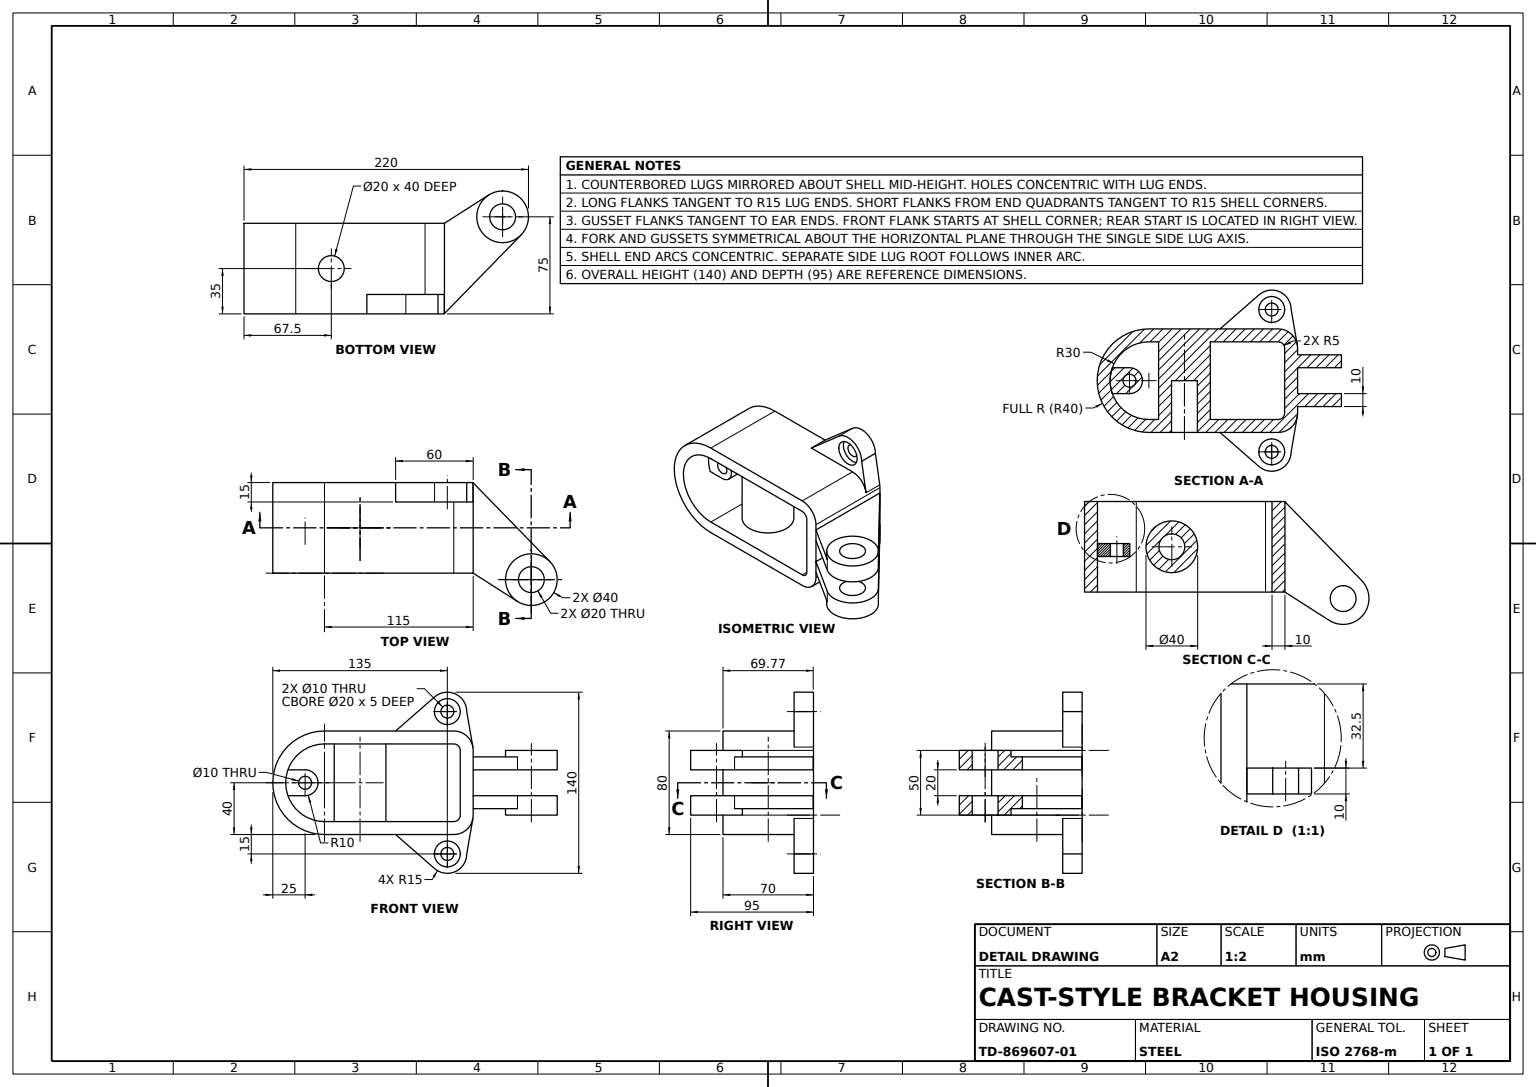
solid
v1 (70,-40,0)
v2 (15,-40,0)
e1 v1 v2 LINE
v3 (-25,0,0)
e2 v3 v2 CIRCLE(AX(P(15,0,0),D(0,0,1),D(1,0,0)),40)
v4 (15,40,0)
e3 v4 v3 CIRCLE(AX(P(15,0,0),D(0,0,1),D(1,0,0)),40)
v5 (70,40,0)
e4 v4 v5 LINE
v6 (100.136986,66.30137,0)
e5 v6 v5 LINE
v7 (125,55,0)
e6 v7 v6 CIRCLE(AX(P(110,55,0),D(0,0,1),D(1,0,0)),15)
v8 (129.77747,27.574177,0)
e7 v7 v8 LINE
v9 (130,25,0)
e8 v8 v9 CIRCLE(AX(P(115,25,0),D(0,0,-1),D(1,0,0)),15)
v10 (130,-25,0)
e9 v9 v10 LINE
v11 (129.77747,-27.574177,0)
e10 v10 v11 CIRCLE(AX(P(115,-25,0),D(0,0,-1),D(1,0,0)),15)
v12 (125,-55,0)
e11 v12 v11 LINE
v13 (100.136986,-66.30137,0)
e12 v12 v13 CIRCLE(AX(P(110,-55,0),D(0,0,-1),D(1,0,0)),15)
e13 v13 v1 LINE
v14 (105,55,0)
v15 (115,55,0)
e14 v14 v15 CIRCLE(AX(P(110,55,0),D(0,0,1),D(1,0,0)),5)
e15 v15 v14 CIRCLE(AX(P(110,55,0),D(0,0,1),D(1,0,0)),5)
v16 (120,25,0)
v17 (120,-25,0)
e16 v16 v17 LINE
v18 (115,30,0)
e17 v18 v16 CIRCLE(AX(P(115,25,0),D(0,0,-1),D(1,0,0)),5)
v19 (15,30,0)
e18 v19 v18 LINE
v20 (-15,0,0)
e19 v19 v20 CIRCLE(AX(P(15,0,0),D(0,0,1),D(1,0,0)),30)
v21 (15,-30,0)
e20 v20 v21 CIRCLE(AX(P(15,0,0),D(0,0,1),D(1,0,0)),30)
v22 (115,-30,0)
e21 v22 v21 LINE
e22 v17 v22 CIRCLE(AX(P(115,-25,0),D(0,0,-1),D(1,0,0)),5)
v23 (115,-55,0)
v24 (105,-55,0)
e23 v23 v24 CIRCLE(AX(P(110,-55,0),D(0,0,-1),D(1,0,0)),5)
e24 v24 v23 CIRCLE(AX(P(110,-55,0),D(0,0,-1),D(1,0,0)),5)
face PLANE(AX(P(0,0,0),D(0,0,1),D(1,0,0))) rev [e1 -e2 -e3 e4 -e5 -e6 e7 e8 e9 e10 -e11 e12 e13] [e14 e15] [-e16 -e17 -e18 e19 e20 -e21 -e22] [-e23 -e24]
v25 (100,55,15)
v26 (120,55,15)
e25 v25 v26 CIRCLE(AX(P(110,55,15),D(0,0,1),D(1,0,0)),10)
v27 (120,55,10)
e26 v26 v27 LINE
v28 (100,55,10)
e27 v28 v27 CIRCLE(AX(P(110,55,10),D(0,0,1),D(1,0,0)),10)
e28 v25 v28 LINE
face CYL(AX(P(110,55,15),D(0,0,-1),D(-1,0,0)),10) rev [e25 e26 -e27 -e28]
v29 (42.5,30,55)
v30 (42.5,30,15)
e29 v29 v30 CIRCLE(AX(P(42.5,30,35),D(0,-1,0),D(0,0,1)),20)
v31 (42.5,-30,15)
e30 v30 v31 LINE
v32 (42.5,-30,55)
e31 v31 v32 CIRCLE(AX(P(42.5,-30,35),D(0,1,0),D(0,0,-1)),20)
e32 v29 v32 LINE
face CYL(AX(P(42.5,86.568542,35),D(0,-1,0),D(0,0,-1)),20) [e29 e30 e31 -e32]
v33 (130,-25,70)
v34 (115,-40,70)
e33 v33 v34 CIRCLE(AX(P(115,-25,70),D(0,0,-1),D(1,0,0)),15)
v35 (115,-40,15)
e34 v34 v35 LINE
v36 (129.77747,-27.574177,15)
e35 v36 v35 CIRCLE(AX(P(115,-25,15),D(0,0,-1),D(1,0,0)),15)
e36 v36 v11 LINE
e37 v33 v10 LINE
face CYL(AX(P(115,-25,70),D(0,0,-1),D(-1,0,0)),15) [e33 e34 -e35 e36 -e10 -e37]
v37 (189.316428,-10,61.034332)
v38 (130,-10,0.228119)
e38 v37 v38 LINE
v39 (189.316428,-20,61.034332)
e39 v39 v37 LINE
v40 (130,-20,0.228119)
e40 v39 v40 LINE
e41 v40 v38 LINE
face PLANE(AX(P(66.498013,-20,-64.868776),D(0.715821408,0,-0.698283403),D(-0.698283403,0,-0.715821408))) [-e38 -e39 e40 e41]
v41 (175,25,55)
v42 (175,25,95)
e42 v41 v42 CIRCLE(AX(P(175,25,75),D(0,1,0),D(0,0,1)),20)
v43 (175,20,55)
e43 v41 v43 LINE
v44 (164.238039,20,91.857645)
e44 v43 v44 CIRCLE(AX(P(175,20,75),D(0,1,0),D(0,0,1)),20)
v45 (164.238039,10,91.857645)
e45 v44 v45 LINE
v46 (175,10,95)
e46 v45 v46 CIRCLE(AX(P(175,10,75),D(0,1,0),D(0,0,1)),20)
e47 v42 v46 LINE
face CYL(AX(P(175,25,75),D(0,-1,0),D(0,0,-1)),20) [-e42 e43 e44 e45 e46 -e47]
e48 v42 v41 CIRCLE(AX(P(175,25,75),D(0,1,0),D(0,0,1)),20)
v47 (175,25,85)
v48 (175,25,65)
e49 v47 v48 CIRCLE(AX(P(175,25,75),D(0,1,0),D(0,0,1)),10)
e50 v48 v47 CIRCLE(AX(P(175,25,75),D(0,1,0),D(0,0,1)),10)
face PLANE(AX(P(0,25,0),D(0,1,0),D(0,0,1))) [e48 e42] [-e49 -e50]
v49 (100,-55,15)
v50 (100,-55,10)
e51 v49 v50 LINE
v51 (120,-55,15)
e52 v51 v49 CIRCLE(AX(P(110,-55,15),D(0,0,-1),D(1,0,0)),10)
v52 (120,-55,10)
e53 v51 v52 LINE
e54 v52 v50 CIRCLE(AX(P(110,-55,10),D(0,0,-1),D(1,0,0)),10)
face CYL(AX(P(110,-55,15),D(0,0,-1),D(-1,0,0)),10) rev [-e51 -e52 e53 e54]
v53 (105,-55,10)
e55 v53 v24 LINE
v54 (115,-55,10)
e56 v54 v23 LINE
e57 v54 v53 CIRCLE(AX(P(110,-55,10),D(0,0,1),D(1,0,0)),5)
face CYL(AX(P(110,-55,70),D(0,0,-1),D(-1,0,0)),5) rev [e55 e24 -e56 e57]
v55 (-15,0,70)
e58 v55 v20 LINE
v56 (15,-30,70)
e59 v55 v56 CIRCLE(AX(P(15,0,70),D(0,0,1),D(1,0,0)),30)
e60 v56 v21 LINE
face CYL(AX(P(15,0,70),D(0,0,-1),D(-1,0,0)),30) rev [-e20 -e58 e59 e60]
v57 (129.77747,27.574177,15)
e61 v57 v8 LINE
v58 (115,40,15)
e62 v58 v57 CIRCLE(AX(P(115,25,15),D(0,0,-1),D(1,0,0)),15)
v59 (115,40,70)
e63 v59 v58 LINE
v60 (130,25,70)
e64 v59 v60 CIRCLE(AX(P(115,25,70),D(0,0,-1),D(1,0,0)),15)
e65 v60 v9 LINE
face CYL(AX(P(115,25,70),D(0,0,-1),D(-1,0,0)),15) [-e61 -e62 -e63 e64 e65 -e8]
v61 (42.5,0,25)
v62 (42.5,0,45)
e66 v61 v62 CIRCLE(AX(P(42.5,0,35),D(0,1,0),D(0,0,1)),10)
e67 v62 v61 CIRCLE(AX(P(42.5,0,35),D(0,1,0),D(0,0,1)),10)
face PLANE(AX(P(0,0,0),D(0,1,0),D(0,0,1))) rev [-e66 -e67]
v63 (105,55,10)
e68 v63 v14 LINE
v64 (115,55,10)
e69 v64 v63 CIRCLE(AX(P(110,55,10),D(0,0,-1),D(1,0,0)),5)
e70 v64 v15 LINE
face CYL(AX(P(110,55,70),D(0,0,-1),D(-1,0,0)),5) rev [-e14 -e68 -e69 e70]
v65 (125,-55,15)
e71 v65 v36 LINE
e72 v65 v12 LINE
face PLANE(AX(P(130.617297,-22.753016,15),D(-0.985164654,0.171611782,0),D(-0.171611782,-0.985164654,0))) rev [-e36 -e71 e72 e11]
v66 (70,-40,15)
e73 v66 v1 LINE
v67 (100.136986,-66.30137,15)
e74 v67 v13 LINE
e75 v67 v66 LINE
face PLANE(AX(P(10.448489,11.972227,15),D(-0.657534247,-0.753424658,0),D(0.753424658,-0.657534247,0))) [e73 -e13 -e74 e75]
e76 v26 v25 CIRCLE(AX(P(110,55,15),D(0,0,1),D(1,0,0)),10)
v68 (100.136986,66.30137,15)
v69 (70,40,15)
e77 v68 v69 LINE
e78 v69 v58 LINE
v70 (125,55,15)
e79 v70 v57 LINE
e80 v70 v68 CIRCLE(AX(P(110,55,15),D(0,0,1),D(1,0,0)),15)
face PLANE(AX(P(0,0,15),D(0,0,1),D(1,0,0))) [-e25 -e76] [e77 e78 e62 -e79 e80]
v71 (42.5,-40,45)
e81 v71 v62 LINE
v72 (42.5,-40,25)
e82 v72 v61 LINE
e83 v72 v71 CIRCLE(AX(P(42.5,-40,35),D(0,-1,0),D(0,0,-1)),10)
face CYL(AX(P(42.5,-86.568542,35),D(0,1,0),D(0,0,1)),10) rev [e81 e67 -e82 e83]
v73 (175,10,85)
v74 (175,10,65)
e84 v73 v74 CIRCLE(AX(P(175,10,75),D(0,1,0),D(0,0,1)),10)
e85 v74 v73 CIRCLE(AX(P(175,10,75),D(0,1,0),D(0,0,1)),10)
v75 (189.316428,10,61.034332)
v76 (130,10,0.228119)
e86 v75 v76 LINE
e87 v46 v75 CIRCLE(AX(P(175,10,75),D(0,1,0),D(0,0,1)),20)
v77 (130,10,70)
e88 v45 v77 LINE
e89 v76 v77 LINE
face PLANE(AX(P(0,10,0),D(0,1,0),D(0,0,1))) rev [e84 e85] [-e86 -e87 -e46 e88 -e89]
v78 (115,-30,70)
e90 v78 v22 LINE
v79 (120,-25,70)
e91 v79 v78 CIRCLE(AX(P(115,-25,70),D(0,0,-1),D(1,0,0)),5)
e92 v79 v17 LINE
face CYL(AX(P(115,-25,70),D(0,0,-1),D(-1,0,0)),5) rev [-e90 -e91 e92 e22]
v80 (189.316428,20,61.034332)
e93 v80 v75 LINE
e94 v80 v43 CIRCLE(AX(P(175,20,75),D(0,1,0),D(0,0,1)),20)
face CYL(AX(P(175,25,75),D(0,-1,0),D(0,0,-1)),20) [e87 -e93 e94 -e43 -e48 e47]
e95 v27 v28 CIRCLE(AX(P(110,55,10),D(0,0,1),D(1,0,0)),10)
face CYL(AX(P(110,55,15),D(0,0,-1),D(-1,0,0)),10) rev [e28 -e95 -e26 e76]
v81 (-25,0,70)
e96 v81 v3 LINE
v82 (15,-40,70)
e97 v82 v2 LINE
e98 v81 v82 CIRCLE(AX(P(15,0,70),D(0,0,1),D(1,0,0)),40)
face CYL(AX(P(15,0,70),D(0,0,-1),D(-1,0,0)),40) [e96 e2 -e97 -e98]
v83 (164.238039,-10,91.857645)
v84 (130,-10,70)
e99 v83 v84 LINE
v85 (130,-20,70)
e100 v85 v84 LINE
v86 (164.238039,-20,91.857645)
e101 v86 v85 LINE
e102 v86 v83 LINE
face PLANE(AX(P(5.892704,-20,-9.230391),D(0.538098029,0,-0.842882264),D(-0.842882264,0,-0.538098029))) rev [e99 -e100 -e101 e102]
e103 v71 v72 CIRCLE(AX(P(42.5,-40,35),D(0,-1,0),D(0,0,-1)),10)
face CYL(AX(P(42.5,-86.568542,35),D(0,1,0),D(0,0,1)),10) rev [-e81 e103 e82 e66]
v87 (120,25,70)
e104 v87 v79 LINE
e105 v87 v16 LINE
face PLANE(AX(P(120,0,70),D(1,0,0),D(0,0,-1))) rev [e16 -e92 -e104 e105]
e106 v49 v51 CIRCLE(AX(P(110,-55,15),D(0,0,-1),D(1,0,0)),10)
e107 v50 v52 CIRCLE(AX(P(110,-55,10),D(0,0,-1),D(1,0,0)),10)
face CYL(AX(P(110,-55,15),D(0,0,-1),D(-1,0,0)),10) rev [-e106 e51 e107 -e53]
e108 v35 v66 LINE
e109 v34 v82 LINE
face PLANE(AX(P(0,-40,70),D(0,-1,0),D(1,0,0))) [-e103 -e83] [-e1 -e73 -e108 -e34 e109 e97]
v88 (15,40,70)
e110 v88 v59 LINE
e111 v69 v5 LINE
e112 v88 v4 LINE
face PLANE(AX(P(0,40,70),D(0,1,0),D(-1,0,0))) [e110 e63 -e78 e111 -e4 -e112]
e113 v65 v67 CIRCLE(AX(P(110,-55,15),D(0,0,-1),D(1,0,0)),15)
face CYL(AX(P(110,-55,15),D(0,0,-1),D(-1,0,0)),15) [e113 e74 -e12 -e72]
e114 v78 v56 LINE
e115 v32 v31 CIRCLE(AX(P(42.5,-30,35),D(0,1,0),D(0,0,-1)),20)
face PLANE(AX(P(0,-30,70),D(0,-1,0),D(0,0,-1))) rev [e21 -e60 -e114 e90] [-e31 -e115]
v89 (175,-25,85)
v90 (175,-10,85)
e116 v89 v90 LINE
v91 (175,-25,65)
e117 v91 v89 CIRCLE(AX(P(175,-25,75),D(0,1,0),D(0,0,1)),10)
v92 (175,-10,65)
e118 v91 v92 LINE
e119 v92 v90 CIRCLE(AX(P(175,-10,75),D(0,1,0),D(0,0,1)),10)
face CYL(AX(P(175,-25,75),D(0,1,0),D(0,0,1)),10) rev [-e116 -e117 e118 e119]
v93 (175,-25,55)
v94 (175,-20,55)
e120 v93 v94 LINE
v95 (175,-25,95)
e121 v93 v95 CIRCLE(AX(P(175,-25,75),D(0,1,0),D(0,0,1)),20)
v96 (175,-10,95)
e122 v95 v96 LINE
e123 v83 v96 CIRCLE(AX(P(175,-10,75),D(0,1,0),D(0,0,1)),20)
e124 v94 v86 CIRCLE(AX(P(175,-20,75),D(0,1,0),D(0,0,1)),20)
face CYL(AX(P(175,-25,75),D(0,1,0),D(0,0,1)),20) [-e120 e121 e122 -e123 -e102 -e124]
v97 (130,20,0.228119)
e125 v80 v97 LINE
v98 (130,20,70)
e126 v97 v98 LINE
e127 v44 v98 LINE
face PLANE(AX(P(0,20,0),D(0,1,0),D(0,0,1))) [-e44 -e94 e125 e126 -e127]
e128 v85 v40 LINE
e129 v85 v33 LINE
e130 v60 v98 LINE
e131 v97 v76 LINE
e132 v77 v84 LINE
e133 v84 v38 LINE
face PLANE(AX(P(130,0,70),D(1,0,0),D(0,0,-1))) [-e128 e129 e37 -e9 -e65 e130 -e126 e131 e89 e132 e133 -e41]
e134 v90 v92 CIRCLE(AX(P(175,-10,75),D(0,1,0),D(0,0,1)),10)
e135 v89 v91 CIRCLE(AX(P(175,-25,75),D(0,1,0),D(0,0,1)),10)
face CYL(AX(P(175,-25,75),D(0,1,0),D(0,0,1)),10) rev [e116 e134 -e118 -e135]
v99 (115,30,70)
e136 v99 v87 CIRCLE(AX(P(115,25,70),D(0,0,-1),D(1,0,0)),5)
e137 v99 v18 LINE
face CYL(AX(P(115,25,70),D(0,0,-1),D(-1,0,0)),5) rev [-e136 e137 e17 -e105]
e138 v68 v6 LINE
face PLANE(AX(P(10.448489,-11.972227,15),D(0.657534247,-0.753424658,0),D(0.753424658,0.657534247,0))) rev [e138 e5 -e111 -e77]
face PLANE(AX(P(0,0,15),D(0,0,1),D(1,0,0))) [e108 -e75 -e113 e71 e35] [e52 e106]
e139 v39 v94 CIRCLE(AX(P(175,-20,75),D(0,1,0),D(0,0,1)),20)
face PLANE(AX(P(0,-20,0),D(0,-1,0),D(0,0,1))) [-e40 e139 e124 e101 e128]
e140 v96 v37 CIRCLE(AX(P(175,-10,75),D(0,1,0),D(0,0,1)),20)
face PLANE(AX(P(0,-10,0),D(0,-1,0),D(0,0,1))) rev [-e119 -e134] [-e99 e123 e140 e38 -e133]
v100 (15,30,70)
e141 v100 v55 CIRCLE(AX(P(15,0,70),D(0,0,1),D(1,0,0)),30)
e142 v100 v99 LINE
e143 v98 v77 LINE
e144 v88 v81 CIRCLE(AX(P(15,0,70),D(0,0,1),D(1,0,0)),40)
face PLANE(AX(P(0,0,70),D(0,0,1),D(1,0,0))) [e91 e114 -e59 -e141 e142 e136 e104] [-e129 e100 -e132 -e143 -e130 -e64 -e110 e144 e98 -e109 -e33]
e145 v100 v19 LINE
face CYL(AX(P(15,0,70),D(0,0,-1),D(-1,0,0)),30) rev [e141 e58 -e19 -e145]
e146 v47 v73 LINE
e147 v48 v74 LINE
face CYL(AX(P(175,25,75),D(0,-1,0),D(0,0,-1)),10) rev [-e146 e49 e147 -e84]
e148 v95 v93 CIRCLE(AX(P(175,-25,75),D(0,1,0),D(0,0,1)),20)
face PLANE(AX(P(0,-25,0),D(0,-1,0),D(0,0,1))) [e135 e117] [-e148 -e121]
e149 v70 v7 LINE
face CYL(AX(P(110,55,15),D(0,0,-1),D(-1,0,0)),15) [-e80 e149 e6 -e138]
e150 v63 v64 CIRCLE(AX(P(110,55,10),D(0,0,-1),D(1,0,0)),5)
face CYL(AX(P(110,55,70),D(0,0,-1),D(-1,0,0)),5) rev [-e15 -e70 -e150 e68]
face CYL(AX(P(15,0,70),D(0,0,-1),D(-1,0,0)),40) [e3 -e96 -e144 e112]
face PLANE(AX(P(5.892704,20,-9.230391),D(-0.538098029,0,0.842882264),D(0.842882264,0,0.538098029))) [-e88 -e45 e127 e143]
face PLANE(AX(P(66.498013,20,-64.868776),D(-0.715821408,0,0.698283403),D(0.698283403,0,0.715821408))) rev [-e131 -e125 e93 e86]
e151 v53 v54 CIRCLE(AX(P(110,-55,10),D(0,0,1),D(1,0,0)),5)
face CYL(AX(P(110,-55,70),D(0,0,-1),D(-1,0,0)),5) rev [e56 e23 -e55 e151]
face PLANE(AX(P(0,0,10),D(0,0,1),D(1,0,0))) [-e54 -e107] [-e151 -e57]
face PLANE(AX(P(0,0,10),D(0,0,1),D(1,0,0))) [e27 e95] [e150 e69]
face CYL(AX(P(175,-25,75),D(0,1,0),D(0,0,1)),20) [e39 -e140 -e122 e148 e120 -e139]
e152 v30 v29 CIRCLE(AX(P(42.5,30,35),D(0,-1,0),D(0,0,1)),20)
face PLANE(AX(P(0,30,70),D(0,1,0),D(0,0,1))) rev [-e29 -e152] [-e137 -e142 e145 e18]
face CYL(AX(P(175,25,75),D(0,-1,0),D(0,0,-1)),10) rev [e50 e146 -e85 -e147]
face PLANE(AX(P(130.617297,22.753016,15),D(0.985164654,0.171611782,0),D(-0.171611782,0.985164654,0))) [-e149 e79 e61 -e7]
face CYL(AX(P(42.5,86.568542,35),D(0,-1,0),D(0,0,-1)),20) [-e30 e152 e32 e115]
solid
v101 (-15,0,32.5)
v102 (-13.284271,-10,32.5)
e153 v101 v102 CIRCLE(AX(P(15,0,32.5),D(0,0,1),D(1,0,0)),30)
v103 (-13.284271,-10,42.5)
e154 v103 v102 LINE
v104 (-15,0,42.5)
e155 v104 v103 CIRCLE(AX(P(15,0,42.5),D(0,0,1),D(1,0,0)),30)
e156 v104 v101 LINE
face CYL(AX(P(15,0,42.5),D(0,0,-1),D(-1,0,0)),30) [e153 -e154 -e155 e156]
v105 (-13.284271,10,42.5)
e157 v105 v104 CIRCLE(AX(P(15,0,42.5),D(0,0,1),D(1,0,0)),30)
v106 (-13.284271,10,32.5)
e158 v105 v106 LINE
e159 v106 v101 CIRCLE(AX(P(15,0,32.5),D(0,0,1),D(1,0,0)),30)
face CYL(AX(P(15,0,42.5),D(0,0,-1),D(-1,0,0)),30) [-e157 e158 e159 -e156]
v107 (0,10,32.5)
e160 v107 v106 LINE
v108 (0,10,42.5)
e161 v108 v105 LINE
e162 v108 v107 LINE
face PLANE(AX(P(0,10,42.5),D(0,-1,0),D(0,0,-1))) rev [e160 -e158 -e161 e162]
v109 (-5,0,42.5)
v110 (-5,0,32.5)
e163 v109 v110 LINE
v111 (5,0,32.5)
e164 v111 v110 CIRCLE(AX(P(0,0,32.5),D(0,0,1),D(1,0,0)),5)
v112 (5,0,42.5)
e165 v112 v111 LINE
e166 v112 v109 CIRCLE(AX(P(0,0,42.5),D(0,0,1),D(1,0,0)),5)
face CYL(AX(P(0,0,42.5),D(0,0,-1),D(-1,0,0)),5) rev [e163 -e164 -e165 e166]
v113 (0,-10,32.5)
e167 v113 v102 LINE
v114 (0,-10,42.5)
e168 v114 v113 LINE
e169 v114 v103 LINE
face PLANE(AX(P(0,-10,42.5),D(0,-1,0),D(0,0,-1))) [e154 -e167 -e168 e169]
e170 v110 v111 CIRCLE(AX(P(0,0,32.5),D(0,0,1),D(1,0,0)),5)
e171 v109 v112 CIRCLE(AX(P(0,0,42.5),D(0,0,1),D(1,0,0)),5)
face CYL(AX(P(0,0,42.5),D(0,0,-1),D(-1,0,0)),5) rev [-e170 -e163 e171 e165]
e172 v113 v107 CIRCLE(AX(P(0,0,32.5),D(0,0,1),D(1,0,0)),10)
e173 v114 v108 CIRCLE(AX(P(0,0,42.5),D(0,0,1),D(1,0,0)),10)
face CYL(AX(P(0,0,42.5),D(0,0,-1),D(-1,0,0)),10) [e172 -e162 -e173 e168]
face PLANE(AX(P(0,0,42.5),D(0,0,1),D(1,0,0))) [e173 e161 e157 e155 -e169] [-e166 -e171]
face PLANE(AX(P(0,0,32.5),D(0,0,1),D(1,0,0))) rev [e167 -e153 -e159 -e160 -e172] [e170 e164]
